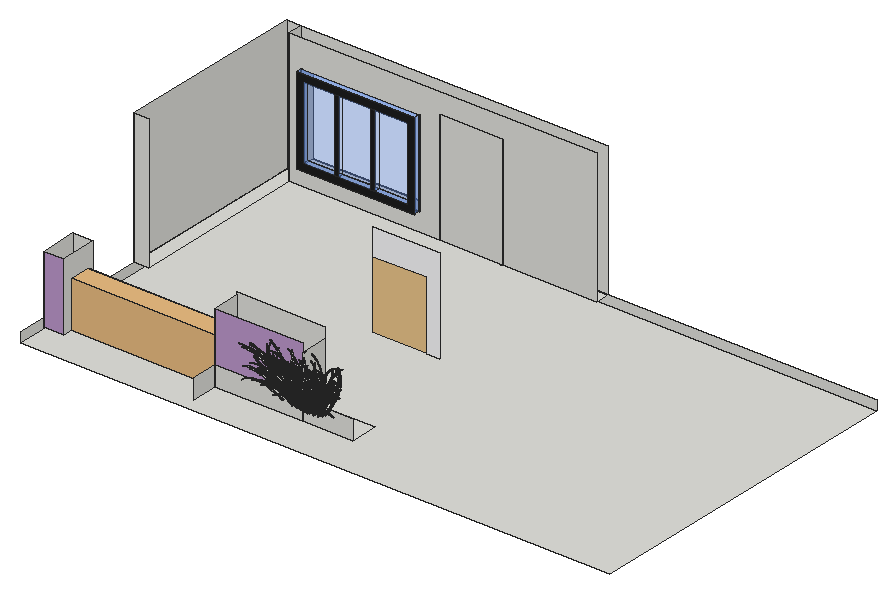
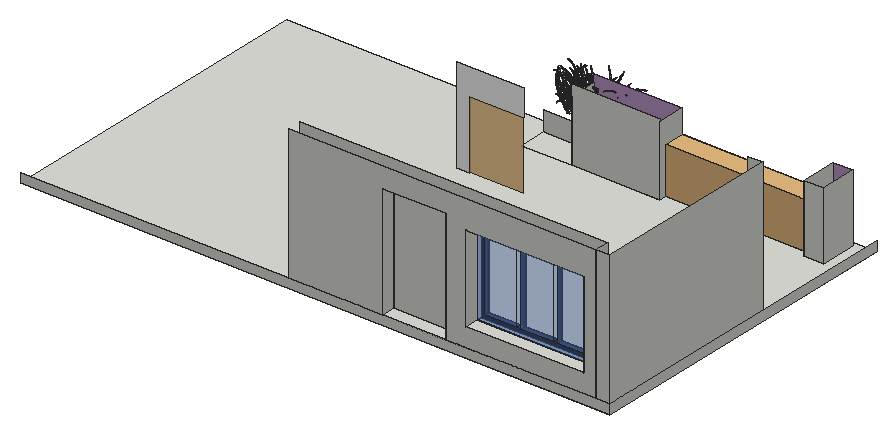
# SketchUp Ruby script. Lengths in inches.
U = 1.inch
M = Sketchup.active_model
def pt(a) = Geom::Point3d.new(a.map { |v| v * U })
def face(e, loops, mat)
  f = e.add_face(loops[0].map { |a| pt(a) })
  loops[1..].each { |l| e.add_face(l.map { |a| pt(a) }).erase! }
  f.material = f.back_material = mat if mat
  f
end
# faces: each face lists its corners as indices into pts; further lists are holes
def faces(e, pts, list, mat = nil) = list.each { |f| face(e, (f[0].is_a?(Array) ? f : [f]).map { |l| l.map { |i| pts[i] } }, mat) }
# xy, xz, yz: faces in a plane at the given z, y or x. An outline is a flat list of corners, or four numbers for a rectangle; further outlines are holes
def ring(l) = l.size == 4 ? [[l[0], l[1]], [l[2], l[1]], [l[2], l[3]], [l[0], l[3]]] : l.each_slice(2).to_a
def flat(e, list, mat, &to3) = list.each { |f| face(e, (f[0].is_a?(Array) ? f : [f]).map { |l| ring(l).map { |u, v| to3.(u, v) } }, mat) }
def xy(e, z, list, mat = nil) = flat(e, list, mat) { |x, y| [x, y, z] }
def xz(e, y, list, mat = nil) = flat(e, list, mat) { |x, z| [x, y, z] }
def yz(e, x, list, mat = nil) = flat(e, list, mat) { |y, z| [x, y, z] }
def lines(e, pts, list) = list.each { |a, b| e.add_line(pt(pts[a]), pt(pts[b])) }
# prism: a flat outline (further loops are holes) pulled along v
def prism(e, loops, v, mat = nil)
  f = face(e, loops, mat); d = Geom::Vector3d.new(v.map { |x| x * U })
  f.pushpull(f.normal.samedirection?(d) ? d.length : -d.length)
end
def box(e, o, s, mat = nil) = prism(e, [[o, [o[0] + s[0], o[1], o[2]], [o[0] + s[0], o[1] + s[1], o[2]], [o[0], o[1] + s[1], o[2]]]], [0, 0, s[2]], mat)
def at(x, y, z, deg = 0) = Geom::Transformation.translation(pt([x, y, z])) * Geom::Transformation.rotation(ORIGIN, Z_AXIS, deg.degrees)
def axes(o, x, y, z) = Geom::Transformation.new([*x, 0, *y, 0, *z, 0, *pt(o).to_a, 1])
def part(name) = M.definitions.add(name)
# library, detail: a bought-in or finely detailed component or shape, given as its bounding box
def library(name, o, s) = part(name).tap { |d| box(d.entities, o, s) }
def detail(e, o, s) = box(e.add_group.entities, o, s)
def put(e, d, t, mat = nil) = e.add_instance(d, t).tap { |i| i.material = mat if mat }
def group(e, t, mat = nil) = e.add_group.tap { |g| g.transformation = t; g.material = mat if mat }.entities
root = M.entities
M.materials.add("[Color L02]").color = [190, 153, 204]
M.materials.add("[Color M08]").color = [30, 30, 30]
M.materials.add("[Formica Laminate Light]").color = [235, 189, 121]
M.materials["[Formica Laminate Light]"].alpha = 0.85
M.materials.add("[Quartz Light Grey]").color = [251, 251, 252]
M.materials.add("[Translucent Glass Blue]").color = [100, 146, 237]
M.materials["[Translucent Glass Blue]"].alpha = 0.42
c1 = part("Group\#1")
xy(c1.entities,0,[[0,0,74.375,3.6875]])
xy(c1.entities,4.39,[[4.39,0,24.03,3.6875],[24.03,0,26.53,3.6875],[26.53,0,47.01,3.6875],[47.01,0,49.38,3.6875],[49.38,0,69.98,3.6875]])
xy(c1.entities,50.55,[[4.39,0,24.03,3.6875],[24.03,0,26.53,3.6875],[26.53,0,47.01,3.6875],[47.01,0,49.38,3.6875],[49.38,0,69.98,3.6875]])
xy(c1.entities,54.9375,[[0,0,74.375,3.6875]])
xz(c1.entities,0,[[[0,0,74.375,54.9375],[4.39,4.39,69.98,50.55]],[24.03,4.39,26.53,50.55],[47.01,4.39,49.38,50.55]],"[Color M08]")
xz(c1.entities,3.6875,[[[0,0,74.375,54.9375],[4.39,4.39,69.98,50.55]]])
xz(c1.entities,3.6875,[[4.39,4.39,24.03,50.55],[26.53,4.39,47.01,50.55],[49.38,4.39,69.98,50.55]],"[Translucent Glass Blue]")
yz(c1.entities,0,[[0,0,3.6875,54.9375]])
yz(c1.entities,4.39,[[0,4.39,3.6875,50.55]])
yz(c1.entities,24.03,[[0,4.39,3.6875,50.55]])
yz(c1.entities,26.53,[[0,4.39,3.6875,50.55]])
yz(c1.entities,47.01,[[0,4.39,3.6875,50.55]])
yz(c1.entities,49.38,[[0,4.39,3.6875,50.55]])
yz(c1.entities,69.98,[[0,4.39,3.6875,50.55]])
yz(c1.entities,74.375,[[0,0,3.6875,54.9375]])
c2 = library("Modern+Gate+1",[0,0,0],[118.11,1.97,78.74])
c3 = part("DOOR12")
g1 = group(c3.entities,at(114.73,28.14,-0.51))
g2 = group(g1,at(0,0,0))
box(g2,[0,0,0],[36,0.5,77.7])
c4 = part("fur_instance\#8")
p = [[-0.25,1.49,0.03],[0.25,-1.49,-0.03],[0.44,-1.47,1.51],[-0.05,1.47,1.57],[0.65,-1.44,3.05],[0.16,1.45,3.11],
  [0.86,-1.42,4.59],[0.38,1.44,4.65],[1.1,-1.39,6.13],[0.62,1.43,6.18],[1.34,-1.35,7.66],[0.875,1.42,7.72],
  [1.6,-1.32,9.19],[1.14,1.41,9.25],[1.88,-1.28,10.72],[1.43,1.41,10.78],[2.18,-1.24,12.25],[1.73,1.41,12.3],
  [2.49,-1.19,13.77],[2.05,1.41,13.82],[2.83,-1.15,15.29],[2.4,1.41,15.34],[3.18,-1.09,16.8],[2.76,1.42,16.85],
  [3.56,-1.03,18.31],[3.14,1.43,18.35],[3.96,-0.97,19.81],[3.55,1.44,19.85],[4.38,-0.91,21.3],[3.99,1.46,21.35],
  [4.84,-0.83,22.78],[4.45,1.48,22.83],[5.32,-0.76,24.26],[4.93,1.51,24.31],[5.82,-0.67,25.73],[5.45,1.54,25.77],
  [6.36,-0.59,27.18],[6,1.57,27.23],[6.93,-0.49,28.625],[6.58,1.61,28.67],[7.54,-0.39,30.05],[7.19,1.66,30.1],
  [8.18,-0.28,31.47],[7.84,1.71,31.51],[8.85,-0.16,32.86],[8.53,1.77,32.9],[9.57,-0.04,34.24],[9.25,1.83,34.27],
  [10.32,0.09,35.59],[10.02,1.9,35.625],[11.12,0.23,36.92],[10.82,1.97,36.95],[11.95,0.38,38.22],[11.67,2.06,38.25],
  [12.84,0.54,39.49],[12.57,2.14,39.52],[13.76,0.71,40.73],[13.51,2.24,40.76],[14.73,0.89,41.93],[14.49,2.34,41.95],
  [15.75,1.08,43.09],[15.52,2.45,43.11],[16.82,1.28,44.2],[16.6,2.5625,44.23],[17.93,1.5,45.27],[17.73,2.68,45.29],
  [19.08,1.73,46.28],[18.9,2.81,46.3],[20.29,1.97,47.24],[20.125,2.93,47.26],[21.53,2.22,48.13],[21.39,3.0625,48.15],
  [22.82,2.5,48.96],[22.7,3.1875,48.98],[24.14,2.8125,49.72],[24.06,3.3,49.73],[25.48,3.27,50.41]]
faces(c4.entities,p,[[0,1,2,3],[3,2,4,5],[5,4,6,7],[7,6,8,9],[9,8,10,11],[11,10,12,13],[13,12,14,15],[15,14,16,17],
  [17,16,18,19],[19,18,20,21],[21,20,22,23],[23,22,24,25],[25,24,26,27],[27,26,28,29],[29,28,30,31],[31,30,32,33],
  [33,32,34,35],[35,34,36,37],[37,36,38,39],[39,38,40,41],[41,40,42,43],[43,42,44,45],[45,44,46,47],[47,46,48,49],
  [49,48,50,51],[51,50,52,53],[53,52,54,55],[55,54,56,57],[57,56,58,59],[59,58,60,61],[61,60,62,63],[63,62,64,65],
  [65,64,66,67],[67,66,68,69],[69,68,70,71],[71,70,72,73],[73,72,74,75],[75,74,76]])
xy(root,-6,[[1.2,32.99,373.22,242.8]])
xy(root,0,[[110.38,49.71,165.8,67.24],[165.8,49.71,197.22,67.24],[1.2,122.8,10.2,242.8],[10.2,233.8,104.9375,242.8],[104.9375,233.8,144.61,242.8],
  [144.61,233.8,204.07,242.8]])
xy(root,11.51,[[18,233.8,92.38,242.8]])
xz(root,44,[[7.2,0,19.58,42.6875]],"[Color L02]")
xz(root,49.71,[[110.38,0,165.8,12.375],[165.8,0,197.22,12.375]])
xz(root,49.71,[[110.38,12.375,165.8,43.9375]],"[Color L02]")
xz(root,67.24,[[110.38,0,165.8,45.75]])
xz(root,67.25,[[7.2,0,19.58,42.6875]])
xz(root,122.8,[[1.2,0,10.2,84]])
xz(root,122.8,[[151.88,13.01,185.45,56.09]],"[Formica Laminate Light]")
xz(root,122.8,[[185.45,13.01,194.19,13.01,194.19,72.94,151.88,72.94,151.88,56.09,185.45,56.09]],"[Quartz Light Grey]")
xz(root,233.8,[[[10.2,0,104.9375,0,104.9375,71.33,144.61,71.33,144.61,0,204.07,0,204.07,84,10.2,84],[18,11.51,92.38,66.45]]])
xz(root,242.8,[[1.2,-6,373.22,0],[1.2,0,10.2,84],[[10.2,0,10.2,84,204.07,84,204.07,0,144.61,0,144.61,71.33,104.9375,71.33,104.9375,0],[18,11.51,92.38,66.45]]])
yz(root,1.2,[[32.99,-6,242.8,0],[122.8,0,242.8,84]])
yz(root,7.2,[[44,0,67.25,42.6875]])
yz(root,10.2,[[233.8,0,242.8,84]])
yz(root,18,[[233.8,11.51,242.8,66.45]])
yz(root,19.58,[[44,0,67.25,42.6875]])
yz(root,92.38,[[233.8,11.51,242.8,66.45]])
yz(root,104.9375,[[233.8,0,242.8,71.33]])
yz(root,110.38,[[32.99,0,49.71,12.375],[49.71,0,67.24,43.9375]])
yz(root,144.61,[[233.8,0,242.8,71.33]])
yz(root,165.8,[[49.71,0,67.24,38.8125]])
put(root,c1,at(17.67,230.11,11.38),"[Translucent Glass Blue]")
put(root,c2,axes([19.58,49.71,0],[0.76881,0,0],[0,6.73905,0],[0,0,0.37275]))
put(root,c3,axes([-21.5,205.66,0.47],[1.10201,0,0],[0,1,0],[0,0,0.91801]))
put(root,c4,axes([157.64,46.96,16.1],[-0.386,-0.06653,-0.25461],[0.24386,-0.13505,0.27151],[-0.38113,0.00133,0.45401]))
put(root,c4,axes([159.27,45.48,16.82],[-0.18851,0.14157,-0.15639],[-0.39353,-0.03374,-0.32881],[-0.37965,-0.016,0.43978]))
put(root,c4,axes([162.18,43.67,18.29],[-0.43293,0.09625,-0.24447],[-0.1572,-0.09955,-0.2799],[-0.35883,-0.05167,0.44054]))
put(root,c4,axes([160.69,44.82,16.96],[-0.27574,0.12477,-0.22934],[-0.32314,-0.06713,-0.27027],[-0.36959,-0.01557,0.42813]))
put(root,c4,axes([158.81,43.86,14.87],[-0.05006,-0.10207,-0.28996],[0.38044,-0.0886,0.33101],[-0.42211,-0.05084,0.35135]))
put(root,c4,axes([158.94,42.64,12.84],[-0.18374,-0.04845,-0.45351],[0.44599,-0.1078,0.07139],[-0.34252,-0.09197,0.36092]))
put(root,c4,axes([160.42,45.39,15.36],[-0.20878,-0.11117,-0.09072],[0.3612,-0.08102,0.32779],[-0.34825,0.00122,0.41485]))
put(root,c4,axes([163.08,45.07,13.92],[-0.31055,-0.01193,-0.33761],[0.04066,-0.12369,0.1649],[-0.38029,0.01052,0.30875]))
put(root,c4,axes([160.48,44.65,13.42],[0.04394,-0.13024,0.05985],[0.31341,-0.01061,0.39141],[-0.40898,-0.00778,0.32218]))
put(root,c4,axes([161.83,43.58,13.6875],[-0.07508,-0.0992,-0.20077],[0.30738,-0.07646,0.33285],[-0.3945,-0.02647,0.31323]))
put(root,c4,axes([162.89,45.5,14.52],[-0.13939,0.10899,-0.32667],[-0.32115,-0.06191,-0.20477],[-0.3674,0.02815,0.31987]))
put(root,c4,axes([165.03,42.97,15.99],[-0.39714,0.04734,-0.28246],[0.005,-0.10962,-0.15138],[-0.30943,-0.04456,0.37988]))
put(root,c4,axes([164.24,43.05,12.79],[-0.18362,0.10871,-0.13495],[-0.21903,-0.03133,-0.32414],[-0.35634,-0.02391,0.28293]))
put(root,c4,axes([165.15,42.98,18.97],[-0.54557,0.03251,-0.20201],[0.04586,-0.12541,-0.20025],[-0.21595,-0.07357,0.50657]))
put(root,c4,axes([164.71,42.8125,13.5625],[-0.25568,-0.00254,-0.35697],[0.17763,-0.10963,0.00665],[-0.34247,-0.04124,0.28506]))
put(root,c4,axes([166.05,42.05,13.58],[-0.31486,0.09259,-0.11403],[-0.14105,-0.04475,-0.34207],[-0.31312,-0.05774,0.2855]))
put(root,c4,axes([164.91,45.21,14.72],[-0.28212,-0.08201,-0.09406],[0.266,-0.09029,0.28696],[-0.29189,0.01469,0.37192]))
put(root,c4,axes([166.08,44.5,12.98],[-0.29855,0.00808,-0.30524],[-0.0548,-0.10838,0.13626],[-0.31854,0.0244,0.27734]))
put(root,c4,axes([160.76,44.36,13.79],[0.31016,-0.00259,0.38704],[-0.06313,0.13066,-0.0838],[-0.40903,-0.00778,0.32222]))
put(root,c4,axes([164.92,46.4375,16.94],[-0.23051,0.11191,-0.31685],[-0.39045,-0.07195,-0.10337],[-0.29068,0.02979,0.41423]))
put(root,c4,axes([160.49,45.06,13.7],[0.32581,-0.02776,0.39303],[0.05892,0.1284,-0.05749],[-0.40202,0.01112,0.3264]))
put(root,c4,axes([164.15,46.29,19.15],[-0.18274,0.13943,-0.18772],[-0.47593,-0.03963,-0.1853],[-0.26085,0.0022,0.49999]))
put(root,c4,axes([166.44,46.55,13.25],[-0.33949,0.04214,-0.33653],[-0.23052,-0.1033,0.15494],[-0.26981,0.05485,0.31268]))
put(root,c4,axes([166.97,42.49,14.88],[-0.34724,0.06528,-0.21301],[-0.08268,-0.08517,-0.19384],[-0.27808,-0.04004,0.3414]))
put(root,c4,axes([166.95,43.37,14.75],[-0.32304,0.04577,-0.2694],[-0.07061,-0.10034,-0.05966],[-0.2877,-0.01212,0.33327]))
put(root,c4,axes([167.03,42.59,13.32],[-0.25974,0.04516,-0.30097],[-0.00971,-0.09244,-0.10665],[-0.32406,-0.02175,0.2573]))
put(root,c4,axes([166.67,44.94,13.94],[-0.29133,-0.07422,-0.0576],[0.18607,-0.07868,0.33898],[-0.29473,0.03905,0.28785]))
put(root,c4,axes([161.59,46.59,13.55],[0.35559,0.04242,0.27246],[-0.08093,0.12348,-0.29504],[-0.3827,0.02932,0.3332]))
put(root,c4,axes([163.75,44.11,14.22],[0.16242,-0.11283,0.20698],[0.24363,0.04343,0.30226],[-0.37838,-0.0072,0.29808]))
put(root,c4,axes([167.625,45.7,14.25],[-0.28817,0.05471,-0.34071],[-0.26689,-0.09171,0.0983],[-0.25825,0.0525,0.29927]))
put(root,c4,axes([162.77,42.82,13.08],[0.30766,-0.02099,0.37745],[-0.13191,0.11603,0.07006],[-0.36824,-0.04435,0.30651]))
put(root,c4,axes([163.49,42.74,13.55],[0.25888,0.0104,0.3784],[-0.20649,0.11618,-0.03214],[-0.36427,-0.04387,0.30321]))
put(root,c4,axes([164.7,43.13,14.08],[0.16846,0.0589,0.28457],[-0.23738,0.09903,-0.21653],[-0.3629,-0.02435,0.28814]))
put(root,c4,axes([168.62,45.28,18.03],[-0.3755,0.08039,-0.23164],[-0.27048,-0.09949,0.00355],[-0.20778,0.0114,0.44394]))
put(root,c4,axes([168.5,44.02,13.4375],[-0.25678,0.03863,-0.30014],[-0.17448,-0.08913,0.07257],[-0.2647,0.03507,0.25852]))
put(root,c4,axes([168.32,41.76,12.89],[-0.22789,0.08786,-0.01217],[-0.19349,-0.01485,-0.3122],[-0.27131,-0.05003,0.24739]))
put(root,c4,axes([166.91,43.51,13.4],[-0.03059,-0.10438,0.0662],[0.26428,-0.01569,0.31222],[-0.32303,0.00894,0.26226]))
put(root,c4,axes([169.49,44.1,17.75],[-0.42254,0.01163,-0.19981],[-0.00309,-0.11957,0.08874],[-0.2162,0.00183,0.41441]))
put(root,c4,axes([168.27,48.74,18.43],[-0.43215,0.08902,-0.30788],[-0.38102,-0.10452,0.19312],[-0.14752,0.06176,0.46105]))
put(root,c4,axes([169.64,41.44,13.6],[-0.29816,0.06259,-0.19264],[-0.02357,-0.06349,-0.24616],[-0.27144,-0.05006,0.2475]))
put(root,c4,axes([169.18,43.32,15.76],[-0.37112,0.02059,-0.19535],[-0.02081,-0.10534,0.02914],[-0.20603,-0.00722,0.37011]))
put(root,c4,axes([168.09,43.94,14.63],[-0.15657,0.0966,-0.22031],[-0.30423,-0.04746,-0.14991],[-0.25757,0.01296,0.32819]))
put(root,c4,axes([167.97,43.42,17.86],[-0.19724,-0.09047,-0.15384],[0.38117,-0.08007,0.17481],[-0.24111,-0.03053,0.4265]))
put(root,c4,axes([169.85,41.07,14.01],[-0.36908,0.02007,-0.29169],[0.20913,-0.08159,-0.23167],[-0.22238,-0.08741,0.29117]))
put(root,c4,axes([169.85,41.33,13.29],[-0.32614,0.05994,-0.13849],[-0.02821,-0.0533,-0.2791],[-0.23245,-0.06242,0.24494]))
put(root,c4,axes([169.91,41.25,13.8],[-0.34932,0.06908,-0.07511],[-0.13386,-0.05643,-0.26374],[-0.20598,-0.06107,0.32017]))
put(root,c4,axes([169.78,42.61,15.59],[-0.34863,-0.00154,-0.1891],[0.07317,-0.10261,0.03563],[-0.20369,-0.0161,0.35644]))
put(root,c4,axes([169.87,42.48,17.1],[-0.34511,-0.02853,-0.21809],[0.21511,-0.10585,0.02098],[-0.21376,-0.03881,0.39707]))
put(root,c4,axes([169.93,44.25,13.14],[-0.31629,-0.04513,-0.06824],[0.10255,-0.07833,0.29233],[-0.21862,0.04444,0.25335]))
put(root,c4,axes([169.74,47.16,19.99],[-0.36805,0.10928,-0.2532],[-0.41126,-0.09135,0.05189],[-0.15824,0.02893,0.50438]))
put(root,c4,axes([169.98,43.43,14.13],[-0.24052,0.06267,-0.23704],[-0.19479,-0.07451,-0.0438],[-0.23299,0.01172,0.29688]))
put(root,c4,axes([168.75,41.1,14.13],[-0.23084,0.07782,0.30984],[-0.44406,0.01645,-0.27357],[-0.1764,-0.10825,0.32179]))
put(root,c4,axes([170.24,46.65,13.37],[-0.41625,0.03099,-0.21789],[-0.1872,-0.09409,0.28454],[-0.14027,0.06925,0.30612]))
put(root,c4,axes([166.47,43.5,12.88],[0.25091,0.0313,0.25191],[-0.08747,0.10068,-0.19535],[-0.32264,0.00893,0.26195]))
put(root,c4,axes([167,42.42,14.32],[0.12427,-0.10416,-0.03859],[0.32395,-0.00562,0.27728],[-0.27031,-0.03893,0.33186]))
put(root,c4,axes([171.02,44.49,14.57],[-0.3086,0.05034,-0.24181],[-0.20464,-0.08701,0.0855],[-0.19079,0.03184,0.32139]))
put(root,c4,axes([170.38,41.4,13.97],[-0.24441,0.08048,0.03855],[-0.24899,-0.02108,-0.25284],[-0.19211,-0.05696,0.29861]))
put(root,c4,axes([169.78,41.6,13.68],[-0.1368,0.08714,0.07099],[-0.29194,0.0044,-0.23828],[-0.21724,-0.04552,0.29232]))
put(root,c4,axes([171.46,43.34,16.88],[-0.32048,0.06541,-0.1942],[-0.20217,-0.0856,-0.02687],[-0.19388,0.00164,0.37162]))
put(root,c4,axes([166.78,41.58,12.83],[0.18986,-0.09113,-0.17624],[0.33239,-0.02217,0.31887],[-0.27181,-0.07299,0.28642]))
put(root,c4,axes([168.86,42.69,14.63],[0.07102,0.09168,0.05994],[-0.29657,0.04404,-0.24731],[-0.26533,-0.01118,0.30735]))
put(root,c4,axes([170.31,42.08,14.04],[-0.12497,-0.06379,-0.15375],[0.25005,-0.064,0.17407],[-0.23753,-0.02139,0.27782]))
put(root,c4,axes([171.67,41.01,14.75],[-0.41058,0.00018,-0.20892],[0.19724,-0.08305,-0.22403],[-0.13275,-0.08676,0.35427]))
put(root,c4,axes([171.1,41.31,14.62],[-0.23306,-0.03008,-0.26598],[0.27876,-0.08125,-0.0141],[-0.20006,-0.05931,0.31097]))
put(root,c4,axes([171.8,42.29,15.24],[-0.28852,-0.02331,-0.15737],[0.13848,-0.0892,0.07157],[-0.183,-0.01446,0.32023]))
put(root,c4,axes([167.25,41.8,12.84],[0.30823,-0.03902,0.28582],[-0.08823,0.08724,0.17487],[-0.29097,-0.05366,0.26531]))
put(root,c4,axes([168.5625,43.35,12.88],[0.16153,-0.06899,0.27824],[0.21116,0.06558,0.0911],[-0.279,0.02137,0.24291]))
put(root,c4,axes([171.59,41.12,13.46],[-0.22838,0.07379,0.032],[-0.22581,-0.02051,-0.23325],[-0.17684,-0.05243,0.27488]))
put(root,c4,axes([172.73,46.18,15.36],[-0.43563,0.03491,-0.17117],[-0.15397,-0.10443,0.2359],[-0.11831,0.04953,0.36974]))
put(root,c4,axes([171.11,40.97,13.06],[-0.20208,-0.01452,-0.30392],[0.29163,-0.06876,-0.06857],[-0.18599,-0.07311,0.24354]))
put(root,c4,axes([172.34,41.02,14.05],[-0.34982,0.0235,-0.15065],[0.06569,-0.07025,-0.19799],[-0.1499,-0.0638,0.28886]))
put(root,c4,axes([169.95,40.66,13.04],[-0.17922,0.07477,0.43016],[-0.56689,0.01723,-0.19414],[-0.11407,-0.13265,0.3666]))
put(root,c4,axes([172.77,40.68,14.05],[-0.45764,0.05432,0.12982],[-0.21881,-0.03654,-0.38115],[-0.09732,-0.11318,0.31278]))
put(root,c4,axes([168.96,42.55,13.19],[0.22902,-0.01797,0.2864],[-0.00674,0.09288,-0.012],[-0.29608,-0.00563,0.23324]))
put(root,c4,axes([168.45,46.55,14.33],[0.07083,-0.10007,0.36045],[0.43741,0.03525,0.07944],[-0.21075,0.06459,0.31363]))
put(root,c4,axes([169.26,41.83,14.54],[0.1081,0.06499,0.23125],[-0.32945,0.06768,-0.13424],[-0.23363,-0.04896,0.31439]))
put(root,c4,axes([172.3,42.71,16.6875],[-0.35427,0.05314,-0.11219],[-0.15409,-0.08687,-0.02981],[-0.12588,-0.01446,0.38393]))
put(root,c4,axes([171.93,41.4375,15.65],[-0.35044,-0.01732,-0.17745],[0.20111,-0.0871,-0.1036],[-0.12561,-0.05988,0.36364]))
put(root,c4,axes([172.63,45.78,16.18],[-0.37487,0.06199,-0.22839],[-0.26657,-0.09041,0.17898],[-0.11778,0.04931,0.3681]))
put(root,c4,axes([168.2,44.75,13.34],[0.28214,-0.0342,0.31004],[0.1649,0.09636,-0.09767],[-0.27864,0.03692,0.27213]))
put(root,c4,axes([172.2,41.3125,14.55],[-0.18407,0.07703,0.07555],[-0.26684,-0.00648,-0.2253],[-0.17849,-0.05292,0.27744]))
put(root,c4,axes([173.11,42.7,16.64],[-0.37418,0.02678,-0.11343],[-0.05032,-0.09585,0.00191],[-0.12302,-0.01413,0.3752]))
put(root,c4,axes([168.31,44.78,13.87],[0.33117,0.01704,0.22685],[0.00751,0.10224,-0.23896],[-0.28243,0.03742,0.27584]))
put(root,c4,axes([171.52,42.68,14.98],[-0.14915,-0.07583,-0.04685],[0.28565,-0.05393,0.1647],[-0.17862,-0.00626,0.32086]))
put(root,c4,axes([170.24,41.61,13.57],[0.06325,-0.08605,-0.06658],[0.28523,-0.01762,0.22613],[-0.22761,-0.03278,0.27944]))
put(root,c4,axes([168.84,41.34,12.97],[0.22308,-0.08573,-0.10956],[0.27059,-0.00586,0.31529],[-0.24902,-0.06687,0.26241]))
put(root,c4,axes([173.32,41.38,16.23],[-0.42092,0.01255,-0.09971],[0.06046,-0.08638,-0.18735],[-0.09421,-0.06736,0.37391]))
put(root,c4,axes([171.33,46.61,13.9],[-0.13523,0.09122,-0.35815],[-0.43675,-0.03907,0.02489],[-0.14051,0.06938,0.30666]))
put(root,c4,axes([169.79,42.1,14.38],[0.15994,-0.09233,0.07552],[0.24761,0.02357,0.23297],[-0.25048,-0.02255,0.29296]))
put(root,c4,axes([172.62,45.13,14.96],[-0.29846,0.07025,-0.23488],[-0.29993,-0.07234,0.12679],[-0.10834,0.04536,0.3386]))
put(root,c4,axes([173.51,40.63,13.61],[-0.42843,0.03035,-0.02391],[-0.02035,-0.0463,-0.33962],[-0.08229,-0.0957,0.26447]))
put(root,c4,axes([172.86,42.01,16.6],[-0.33384,-0.03171,-0.12188],[0.20153,-0.09044,-0.01315],[-0.11031,-0.03659,0.3808]))
put(root,c4,axes([172.2,40.84,13.23],[-0.09713,0.06049,0.23531],[-0.32829,0.03065,-0.18709],[-0.17947,-0.07054,0.23499]))
put(root,c4,axes([169.12,47.28,18.41],[0.11073,0.13384,-0.18532],[-0.52264,0.03311,-0.16808],[-0.15318,0.028,0.48824]))
put(root,c4,axes([166.34,47.86,14.91],[0.45138,-0.02528,0.28457],[0.18854,0.11437,-0.29164],[-0.23265,0.0713,0.34623]))
put(root,c4,axes([171.65,42.1875,15.32],[-0.05453,-0.08389,-0.07082],[0.32107,-0.03698,0.16189],[-0.18296,-0.02316,0.32364]))
put(root,c4,axes([173.88,40.7,13.67],[-0.35966,0.02244,-0.09589],[0.03707,-0.06199,-0.22345],[-0.10538,-0.06887,0.28122]))
put(root,c4,axes([173.95,41.22,15.26],[-0.35295,0.02018,-0.09908],[0.02195,-0.07506,-0.15009],[-0.10994,-0.05241,0.31826]))
put(root,c4,axes([171.71,43.85,14.26],[-0.01057,0.09288,-0.19443],[-0.34342,-0.00855,-0.13723],[-0.17703,0.02954,0.29822]))
put(root,c4,axes([174.21,42.76,16.47],[-0.35258,0.03911,-0.10293],[-0.11378,-0.0889,0.02669],[-0.10118,-0.00433,0.36389]))
put(root,c4,axes([169.65,44.83,13.76],[0.28266,0.07339,-0.0351],[-0.21594,0.06298,-0.31922],[-0.23388,0.04754,0.27103]))
put(root,c4,axes([172.2,41.97,15.72],[-0.06872,-0.07983,-0.11238],[0.33024,-0.04354,0.14283],[-0.17731,-0.03219,0.32936]))
put(root,c4,axes([174.03,45.22,14.72],[-0.42905,0.00809,-0.04494],[-0.02,-0.0986,0.26021],[-0.05535,0.04724,0.33619]))
put(root,c4,axes([169.6,41.55,14.04],[0.2539,-0.08676,0.02919],[0.2281,0.03169,0.26159],[-0.22998,-0.04819,0.30947]))
put(root,c4,axes([173.06,44.55,16.36],[-0.25804,0.08872,-0.18645],[-0.34247,-0.06091,0.05945],[-0.0842,0.0256,0.38442]))
put(root,c4,axes([174.69,44.09,13.2],[-0.34287,0.00812,-0.11784],[-0.07356,-0.07568,0.24887],[-0.10777,0.05321,0.2352]))
put(root,c4,axes([170.97,40.88,13.13],[0.16622,0.02727,0.3366],[-0.34627,0.07103,0.0214],[-0.20135,-0.07914,0.26365]))
put(root,c4,axes([173.55,40.74,14.5],[-0.27609,0.07627,0.23016],[-0.39761,-0.0206,-0.2181],[-0.07922,-0.09579,0.36592]))
put(root,c4,axes([172.875,41.83,15.75],[-0.0678,-0.07804,-0.1102],[0.32302,-0.04274,0.13956],[-0.17349,-0.0315,0.32227]))
put(root,c4,axes([168.8125,41.45,15.3],[0.31264,-0.09597,-0.12302],[0.35367,0.021,0.30617],[-0.1988,-0.08462,0.3831]))
put(root,c4,axes([174.13,43.47,15.33],[-0.24814,0.0704,-0.16557],[-0.26457,-0.0617,0.03798],[-0.104,0.01901,0.3315]))
put(root,c4,axes([172.48,46.46,19.32],[-0.07191,0.1327,-0.23744],[-0.52609,-0.01221,-0.04844],[-0.10427,0.0317,0.47602]))
put(root,c4,axes([168.73,40.86,13.24],[0.40722,0.00264,0.36656],[-0.35604,0.08593,0.25535],[-0.19065,-0.11699,0.34779]))
put(root,c4,axes([173.55,47.33,13.7],[-0.19816,0.0922,-0.35366],[-0.44991,-0.04082,0.11704],[-0.07326,0.07526,0.31932]))
put(root,c4,axes([169.8,45.93,13.46],[0.29872,-0.05452,0.31252],[0.28515,0.08249,-0.14377],[-0.19641,0.06019,0.2923]))
put(root,c4,axes([171.61,43.24,15.14],[0.12365,0.08825,-0.04793],[-0.32665,0.03912,-0.16815],[-0.15682,0.00861,0.33505]))
put(root,c4,axes([172.26,41.83,16.11],[0.05303,-0.0911,-0.0966],[0.36078,-0.0166,0.16754],[-0.17062,-0.04257,0.34719]))
put(root,c4,axes([171.19,42.99,14.38],[0.28964,0.01306,0.18071],[-0.04693,0.09137,-0.13987],[-0.22088,0.01111,0.28144]))
put(root,c4,axes([171.57,44.47,13.29],[0.24076,0.07265,-0.13126],[-0.26496,0.04549,-0.26778],[-0.17027,0.05218,0.2534]))
put(root,c4,axes([173.35,40.78,14.1875],[-0.01984,-0.06556,-0.2665],[0.40894,-0.03569,0.06924],[-0.11932,-0.07798,0.31844]))
put(root,c4,axes([172.8,41.05,14.4],[0.09834,-0.0716,-0.18103],[0.33904,-0.01647,0.16768],[-0.14867,-0.06328,0.28649]))
put(root,c4,axes([173.07,40.58,12.82],[0.09654,-0.05683,-0.28804],[0.38343,-0.02683,0.15385],[-0.13936,-0.08552,0.25423]))
put(root,c4,axes([176.8,45.64,13.8125],[-0.40391,0.04329,-0.11566],[-0.16896,-0.07791,0.30684],[0.00175,0.06588,0.28154]))
put(root,c4,axes([171.8,44,14.39],[0.3491,0.00835,0.14021],[-0.00948,0.09444,-0.19712],[-0.17994,0.03003,0.30312]))
put(root,c4,axes([176.375,40.78,14.89],[-0.35191,-0.01191,-0.09793],[0.14916,-0.05711,-0.22709],[-0.01446,-0.07727,0.2853]))
put(root,c4,axes([177.06,40.31,12.57],[-0.38,0.02115,0.06986],[-0.08892,-0.03802,-0.29637],[-0.01477,-0.08877,0.23645]))
put(root,c4,axes([170.34,40.92,13.42],[0.43467,-0.03319,0.15631],[-0.08687,0.06214,0.33103],[-0.15623,-0.09587,0.285]))
put(root,c4,axes([171.99,44.58,14.28],[0.29538,-0.05757,0.22972],[0.24383,0.07765,-0.10278],[-0.14758,0.0381,0.31755]))
put(root,c4,axes([172.83,41,15.33],[0.07915,-0.07689,-0.2978],[0.47199,-0.01375,0.09794],[-0.07833,-0.09471,0.36177]))
put(root,c4,axes([173.49,41.26,16.7],[0.01368,-0.09439,-0.23849],[0.49477,-0.01902,0.04986],[-0.06405,-0.0818,0.4282]))
put(root,c4,axes([172.71,44.35,15.04],[0.29652,0.06496,-0.05614],[-0.24227,0.07155,-0.24525],[-0.14754,0.03809,0.31746]))
put(root,c4,axes([177.09,46.64,14.87],[-0.31402,0.09119,-0.21887],[-0.37063,-0.06354,0.19912],[-0.00167,0.05262,0.37734]))
put(root,c4,axes([175.125,40.37,12.55],[-0.04918,-0.04163,-0.32259],[0.40341,-0.03191,-0.00115],[-0.07797,-0.09067,0.25058]))
put(root,c4,axes([177.15,41.25,17.41],[-0.43769,-0.04742,-0.16933],[0.3246,-0.06798,-0.31013],[0.04734,-0.11092,0.40826]))
put(root,c4,axes([171.2,46.93,14.41],[0.45746,0.03564,-0.00736],[-0.11716,0.0961,-0.37073],[-0.14513,0.07165,0.31673]))
put(root,c4,axes([174.02,40.74,13.94],[0.14036,-0.06694,-0.1901],[0.33996,-0.00392,0.15825],[-0.10719,-0.07005,0.28606]))
put(root,c4,axes([178.67,49.14,15.71],[-0.5147,0.07524,-0.08821],[-0.24852,-0.11027,0.33949],[0.06923,0.05849,0.44716]))
put(root,c4,axes([172.7,43.89,13.98],[0.35184,0.0053,0.10105],[-0.00269,0.08864,-0.20794],[-0.13558,0.035,0.29171]))
put(root,c4,axes([175.76,44.47,13.59],[-0.03936,-0.07815,0.28453],[0.38096,-0.00792,0.05715],[-0.05707,0.05863,0.24876]))
put(root,c4,axes([175.28,43.46,15.95],[0.08731,0.0916,-0.14583],[-0.36918,0.02597,-0.09333],[-0.0745,0.02265,0.3401]))
put(root,c4,axes([177.85,45.82,17.18],[-0.30552,0.1021,-0.1373],[-0.38181,-0.06496,0.1702],[0.03985,0.02792,0.43212]))
put(root,c4,axes([178.01,40.69,14.65],[-0.31735,0.04136,0.19718],[-0.26282,-0.04709,-0.18031],[0.0358,-0.08387,0.30871]))
put(root,c4,axes([172.67,45.06,14.17],[0.38252,-0.03344,0.15739],[0.14691,0.09174,-0.20505],[-0.10492,0.04393,0.32791]))
put(root,c4,axes([177.72,40.36,13],[-0.31093,-0.02387,-0.1306],[0.20536,-0.03341,-0.26143],[0.04259,-0.0856,0.22729]))
put(root,c4,axes([175.25,46.13,14.05],[0.08818,-0.09101,0.3412],[0.4439,0.01826,-0.03451],[-0.06744,0.06928,0.29396]))
put(root,c4,axes([176.73,40.55,13.94],[-0.0525,0.05846,0.24565],[-0.37999,0.00339,-0.03551],[-0.01452,-0.07755,0.28633]))
put(root,c4,axes([177.54,44.18,13.18],[-0.14177,0.07254,-0.25278],[-0.34278,-0.02095,0.11528],[0.00148,0.05582,0.23853]))
put(root,c4,axes([179,44,13.36],[-0.36167,0.0062,0.08214],[0.04865,-0.07708,0.2642],[0.0571,0.05256,0.23747]))
put(root,c4,axes([179.01,47.15,14.64],[-0.35769,0.08811,-0.2147],[-0.34777,-0.05842,0.3114],[0.07806,0.07185,0.32464]))
put(root,c4,axes([173.99,45.86,16.66],[0.33061,0.07661,-0.18493],[-0.3445,0.0789,-0.22797],[-0.06153,0.05251,0.37373]))
put(root,c4,axes([174.74,44.74,13.75],[0.24228,-0.06432,0.25438],[0.31408,0.04982,-0.16011],[-0.05911,0.06072,0.25764]))
put(root,c4,axes([178.36,41.31,16.58],[-0.24785,-0.06883,-0.12708],[0.35282,-0.04718,-0.16961],[0.06345,-0.07216,0.37439]))
put(root,c4,axes([174.86,40.49,13.53],[0.25603,0.0373,0.32811],[-0.42095,0.04032,0.20029],[-0.01865,-0.11207,0.29851]))
put(root,c4,axes([175.89,40.54,13.8],[0.16296,0.04721,0.22549],[-0.34749,0.03469,0.10404],[-0.01452,-0.07759,0.28649]))
put(root,c4,axes([180.48,40.61,14.05],[-0.45852,-0.00131,0.19527],[-0.13526,-0.06032,-0.3321],[0.12869,-0.10984,0.30067]))
put(root,c4,axes([177.04,41.24,16.58],[-0.01123,-0.08332,-0.2137],[0.44411,-0.00764,-0.03766],[0.02499,-0.07541,0.38189]))
put(root,c4,axes([175.58,43.6,14.66],[0.30236,0.04379,-0.09951],[-0.20093,0.07123,-0.19978],[-0.04678,0.03993,0.28415]))
put(root,c4,axes([175.53,40.68,14.38],[0.38609,-0.01064,0.08267],[-0.06869,0.06311,0.24321],[-0.06418,-0.0776,0.29644]))
put(root,c4,axes([175.99,40.5625,14.07],[0.28598,0.04146,0.21691],[-0.33345,0.0527,0.18368],[-0.01662,-0.08881,0.3279]))
put(root,c4,axes([180.72,45.08,13.63],[-0.39009,0.00001,0.17989],[0.11673,-0.09339,0.26452],[0.12739,0.05425,0.27393]))
put(root,c4,axes([178.75,40.46,13.53],[-0.10011,-0.04974,-0.33937],[0.44799,-0.00922,-0.12015],[0.05247,-0.10545,0.28001]))
put(root,c4,axes([179.55,43.21,14.96],[-0.10507,0.08918,-0.12433],[-0.34324,-0.0157,0.10495],[0.06162,0.01736,0.32061]))
put(root,c4,axes([180.47,40.4375,12.625],[-0.33711,-0.02831,0.08276],[0.02962,-0.04471,-0.27396],[0.1458,-0.07681,0.22451]))
put(root,c4,axes([180.47,40.43,12.71],[-0.20682,0.0343,0.31491],[-0.35112,-0.03833,-0.09316],[0.1097,-0.09363,0.2563]))
put(root,c4,axes([176.66,40.34,12.83],[0.35366,-0.04446,-0.24533],[0.31386,0.02832,0.27554],[-0.0179,-0.10756,0.28648]))
put(root,c4,axes([176.8,48.63,18.4],[0.37174,0.09535,-0.28424],[-0.4538,0.09446,-0.21654],[-0.00202,0.06354,0.45568]))
put(root,c4,axes([175.99,45.25,14.03],[0.40871,0.01353,-0.09508],[-0.11242,0.08522,-0.30291],[0.0017,0.06379,0.27258]))
put(root,c4,axes([179.15,44.75,13.17],[0.02443,-0.08292,0.29226],[0.3951,-0.01272,-0.06827],[0.06194,0.05701,0.25759]))
put(root,c4,axes([181.64,44.09,13.75],[-0.35273,0.04196,0.09031],[-0.05297,-0.08064,0.28274],[0.1701,0.04176,0.25312]))
put(root,c4,axes([177.23,40.32,12.76],[0.26474,0.04763,0.30423],[-0.42277,0.02745,0.24595],[0.05702,-0.11459,0.30427]))
put(root,c4,axes([177.62,41.64,17.39],[0.24594,-0.08345,-0.13206],[0.36719,0.04951,0.03605],[0.03486,-0.05637,0.41564]))
put(root,c4,axes([180.18,41.08,16.0625],[-0.09618,-0.07807,-0.28185],[0.47437,-0.00607,-0.14936],[0.1023,-0.09773,0.36978]))
put(root,c4,axes([176.91,40.45,13.62],[0.44113,-0.02302,-0.06994],[0.08893,0.04457,0.34406],[-0.01704,-0.10236,0.27264]))
put(root,c4,axes([178.12,40.44,13.52],[0.23527,-0.04244,-0.32893],[0.394,0.0275,0.14606],[0.05245,-0.10542,0.27992]))
put(root,c4,axes([180.26,40.67,14.15],[0.00382,-0.06742,-0.2664],[0.42038,0.00892,-0.07608],[0.08885,-0.08488,0.32117]))
put(root,c4,axes([178.02,40.875,15.1],[0.35472,-0.02474,-0.07799],[0.10815,0.06531,0.16349],[0.02086,-0.06294,0.31878]))
put(root,c4,axes([183.64,41.19,14.76],[-0.43184,-0.01905,0.19526],[-0.03313,-0.08725,-0.23452],[0.19858,-0.08107,0.35788]))
put(root,c4,axes([177.49,46.62,13.25],[0.45836,0.01027,-0.08849],[-0.10185,0.09502,-0.34035],[0.00188,0.07066,0.30193]))
put(root,c4,axes([179.78,41.59,16.6],[0.10145,-0.09013,-0.11364],[0.39229,0.02249,-0.05196],[0.07197,-0.04716,0.38655]))
put(root,c4,axes([180.73,46.58,13.45],[-0.1095,-0.09046,0.35887],[0.44447,-0.05329,-0.02332],[0.14322,0.06099,0.30796]))
put(root,c4,axes([180.28,44.15,14.71],[0.08116,0.08798,-0.24295],[-0.38269,0.03698,0.03722],[0.09609,0.03592,0.31259]))
put(root,c4,axes([177.68,45.9,14.83],[0.37424,0.04762,-0.20255],[-0.2623,0.09553,-0.194],[0.05536,0.04677,0.35755]))
put(root,c4,axes([182.65,40.8,12.66],[-0.2955,-0.04759,0.05689],[0.10271,-0.03925,-0.27706],[0.18824,-0.06882,0.22337]))
put(root,c4,axes([183.3,40.97,13.38],[-0.34689,-0.03727,0.15255],[0.01016,-0.05739,-0.27417],[0.20881,-0.07635,0.24779]))
put(root,c4,axes([181.84,41.15,14.5],[-0.19738,-0.07213,-0.02649],[0.25889,-0.02649,-0.23796],[0.18717,-0.05596,0.28299]))
put(root,c4,axes([179.03,40.84,14.89],[0.2924,-0.04369,-0.15164],[0.22912,0.0571,0.1017],[0.05466,-0.06217,0.32255]))
put(root,c4,axes([178.62,42.04,17.3],[0.25652,-0.07331,-0.12192],[0.31137,0.06059,-0.02207],[0.08765,-0.04331,0.38823]))
put(root,c4,axes([182.37,43.85,13.875],[-0.25567,0.08038,-0.01621],[-0.20899,-0.05022,0.29613],[0.21473,0.03097,0.25145]))
put(root,c4,axes([178.92,44.2,14.8125],[0.35948,0.0263,-0.14389],[-0.16779,0.08884,-0.19639],[0.04806,0.0406,0.31037]))
put(root,c4,axes([185.62,41.03,14.23],[-0.55122,-0.04568,0.13882],[0.04398,-0.07343,-0.44656],[0.23824,-0.12551,0.36685]))
put(root,c4,axes([178.67,42.52,16.41],[0.35862,0.01505,-0.09024],[-0.08668,0.09371,-0.04681],[0.06985,-0.00527,0.35645]))
put(root,c4,axes([181.64,41.48,16.51],[-0.05057,-0.09753,-0.16085],[0.44554,-0.00021,-0.15936],[0.14192,-0.06829,0.40531]))
put(root,c4,axes([179.8,42.4,16.07],[0.28194,0.05371,-0.10033],[-0.22711,0.07651,0.0173],[0.08206,-0.00961,0.35201]))
put(root,c4,axes([181.68,45.48,13.76],[0.05246,0.08979,-0.33029],[-0.42436,0.03943,0.06128],[0.13378,0.05697,0.28766]))
put(root,c4,axes([182.21,44.52,13],[-0.08679,-0.07884,0.29827],[0.35686,-0.05045,-0.06659],[0.17515,0.04299,0.26063]))
put(root,c4,axes([179.89,40.51,13.53],[0.22472,-0.03372,-0.31914],[0.35206,0.04052,0.10698],[0.11243,-0.09597,0.26269]))
put(root,c4,axes([179.72,42.22,16.12],[0.31689,-0.04722,-0.07282],[0.16707,0.07949,-0.07268],[0.09116,-0.01442,0.35009]))
put(root,c4,axes([181.01,46.01,19.44],[0.1873,0.12065,-0.23785],[-0.49336,0.0642,0.05647],[0.13611,0.01881,0.47922]))
put(root,c4,axes([179.34,42.2,16.89],[0.33885,-0.04674,-0.10631],[0.17861,0.085,-0.04154],[0.10561,-0.02658,0.37525]))
put(root,c4,axes([184.57,46.35,13.56],[-0.2918,-0.05708,0.35888],[0.33696,-0.09822,0.09373],[0.21258,0.05218,0.31632]))
put(root,c4,axes([184,41.17,13.4375],[-0.30138,-0.06173,0.11197],[0.11286,-0.04948,-0.29463],[0.25099,-0.06644,0.25091]))
put(root,c4,axes([180.7,42.14,16.2],[0.25106,-0.0703,-0.08348],[0.27319,0.06235,-0.07248],[0.10229,-0.02574,0.36348]))
put(root,c4,axes([179.6875,43.77,15.04],[0.36375,-0.04184,-0.01895],[0.10509,0.08235,-0.23712],[0.093,0.03476,0.30255]))
put(root,c4,axes([182.24,42.75,14.84],[-0.0081,0.09343,-0.13315],[-0.3199,0.01252,0.18833],[0.19355,0.00875,0.28825]))
put(root,c4,axes([180.24,41.61,18.14],[0.3397,-0.08372,-0.25574],[0.43647,0.06671,0.09219],[0.08138,-0.09256,0.48024]))
put(root,c4,axes([185.44,46.52,14.32],[-0.4244,0.02085,0.27353],[0.06726,-0.12155,0.27224],[0.27941,0.0403,0.3272]))
put(root,c4,axes([185.4,45.51,13.8125],[-0.32428,-0.03379,0.34169],[0.23431,-0.10975,0.11115],[0.26016,0.03753,0.30465]))
put(root,c4,axes([180.04,40.8,14.85],[0.45111,0.01178,-0.07295],[-0.01785,0.07208,0.28844],[0.09542,-0.09116,0.34491]))
put(root,c4,axes([181.38,40.64,13.09],[0.25009,-0.01398,-0.2591],[0.22987,0.05125,0.12404],[0.14635,-0.0771,0.22535]))
